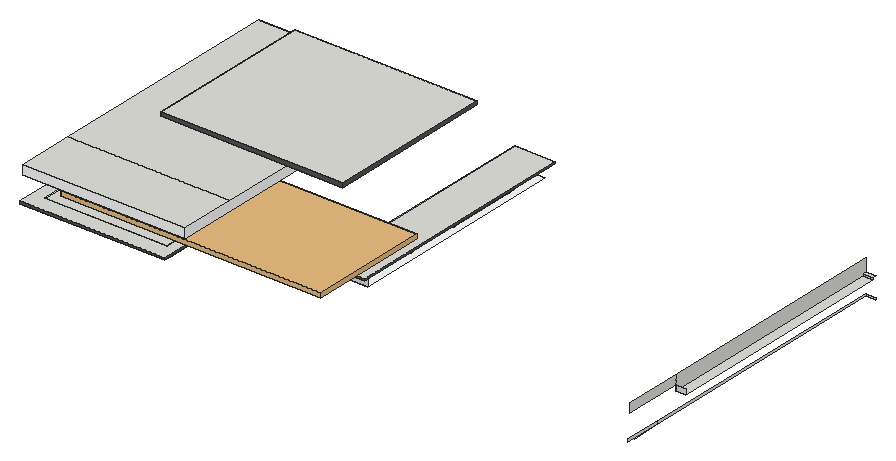
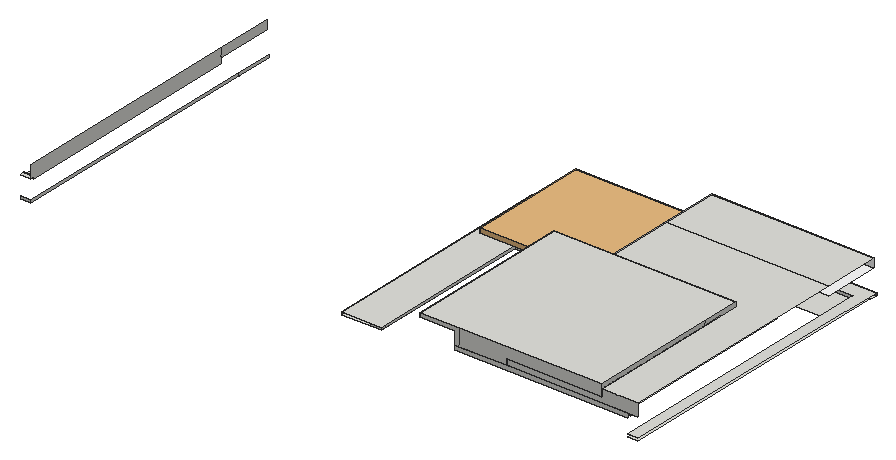
# SketchUp Ruby script. Lengths in inches.
U = 1.inch
M = Sketchup.active_model
def pt(a) = Geom::Point3d.new(a.map { |v| v * U })
def face(e, loops, mat)
  f = e.add_face(loops[0].map { |a| pt(a) })
  loops[1..].each { |l| e.add_face(l.map { |a| pt(a) }).erase! }
  f.material = f.back_material = mat if mat
  f
end
# faces: each face lists its corners as indices into pts; further lists are holes
def faces(e, pts, list, mat = nil) = list.each { |f| face(e, (f[0].is_a?(Array) ? f : [f]).map { |l| l.map { |i| pts[i] } }, mat) }
# xy, xz, yz: faces in a plane at the given z, y or x. An outline is a flat list of corners, or four numbers for a rectangle; further outlines are holes
def ring(l) = l.size == 4 ? [[l[0], l[1]], [l[2], l[1]], [l[2], l[3]], [l[0], l[3]]] : l.each_slice(2).to_a
def flat(e, list, mat, &to3) = list.each { |f| face(e, (f[0].is_a?(Array) ? f : [f]).map { |l| ring(l).map { |u, v| to3.(u, v) } }, mat) }
def xy(e, z, list, mat = nil) = flat(e, list, mat) { |x, y| [x, y, z] }
def xz(e, y, list, mat = nil) = flat(e, list, mat) { |x, z| [x, y, z] }
def yz(e, x, list, mat = nil) = flat(e, list, mat) { |y, z| [x, y, z] }
def lines(e, pts, list) = list.each { |a, b| e.add_line(pt(pts[a]), pt(pts[b])) }
# prism: a flat outline (further loops are holes) pulled along v
def prism(e, loops, v, mat = nil)
  f = face(e, loops, mat); d = Geom::Vector3d.new(v.map { |x| x * U })
  f.pushpull(f.normal.samedirection?(d) ? d.length : -d.length)
end
def box(e, o, s, mat = nil) = prism(e, [[o, [o[0] + s[0], o[1], o[2]], [o[0] + s[0], o[1] + s[1], o[2]], [o[0], o[1] + s[1], o[2]]]], [0, 0, s[2]], mat)
def at(x, y, z, deg = 0) = Geom::Transformation.translation(pt([x, y, z])) * Geom::Transformation.rotation(ORIGIN, Z_AXIS, deg.degrees)
def axes(o, x, y, z) = Geom::Transformation.new([*x, 0, *y, 0, *z, 0, *pt(o).to_a, 1])
def part(name) = M.definitions.add(name)
# library, detail: a bought-in or finely detailed component or shape, given as its bounding box
def library(name, o, s) = part(name).tap { |d| box(d.entities, o, s) }
def detail(e, o, s) = box(e.add_group.entities, o, s)
def put(e, d, t, mat = nil) = e.add_instance(d, t).tap { |i| i.material = mat if mat }
def group(e, t, mat = nil) = e.add_group.tap { |g| g.transformation = t; g.material = mat if mat }.entities
root = M.entities
M.materials.add("[Color M00]").color = [255, 255, 255]
M.materials.add("[Color M06]").color = [86, 86, 86]
c1 = library("Mesh Light\#4",[-0.5,-0.5,-0.1],[1,1,0.2])
c2 = part("Group\#24")
xy(c2.entities,0,[[203.13,95.41,201.58,95.62,200.13,96.22,198.89,97.17,197.9375,98.41,197.34,99.86,197.13,101.41,197.34,102.96,197.9375,104.41,198.89,105.65,200.13,106.61,201.58,107.21,203.13,107.41,204.6875,107.21,206.13,106.61,207.375,105.65,208.33,104.41,208.93,102.96,209.13,101.41,208.93,99.86,208.33,98.41,207.375,97.17,206.13,96.22,204.6875,95.62],[281.57,95.41,280.02,95.62,278.57,96.22,277.33,97.17,276.375,98.41,275.77,99.86,275.57,101.41,275.77,102.96,276.375,104.41,277.33,105.65,278.57,106.61,280.02,107.21,281.57,107.41,283.125,107.21,284.57,106.61,285.8125,105.65,286.77,104.41,287.37,102.96,287.57,101.41,287.37,99.86,286.77,98.41,285.8125,97.17,284.57,96.22,283.125,95.62],[350.95,95.41,349.39,95.62,347.95,96.22,346.7,97.17,345.75,98.41,345.15,99.86,344.95,101.41,345.15,102.96,345.75,104.41,346.7,105.65,347.95,106.61,349.39,107.21,350.95,107.41,352.5,107.21,353.95,106.61,355.1875,105.65,356.14,104.41,356.74,102.96,356.95,101.41,356.74,99.86,356.14,98.41,355.1875,97.17,353.95,96.22,352.5,95.62],[376,162.85,374.44,163.05,373,163.65,371.75,164.6,370.8,165.85,370.2,167.29,370,168.85,370.2,170.4,370.8,171.85,371.75,173.09,373,174.04,374.44,174.64,376,174.85,377.55,174.64,379,174.04,380.24,173.09,381.19,171.85,381.79,170.4,382,168.85,381.79,167.29,381.19,165.85,380.24,164.6,379,163.65,377.55,163.05]],"[Color M00]")
xy(c2.entities,33.4375,[[6,0,4.45,0.2,3,0.8,1.76,1.76,0.8,3,0.2,4.45,0,6,0.2,7.55,0.8,9,1.76,10.24,3,11.2,4.45,11.8,6,12,7.55,11.8,9,11.2,10.24,10.24,11.2,9,11.8,7.55,12,6,11.8,4.45,11.2,3,10.24,1.76,9,0.8,7.55,0.2],[83.125,0,81.57,0.2,80.125,0.8,78.88,1.76,77.93,3,77.33,4.45,77.125,6,77.33,7.55,77.93,9,78.88,10.24,80.125,11.2,81.57,11.8,83.125,12,84.68,11.8,86.125,11.2,87.37,10.24,88.32,9,88.92,7.55,89.125,6,88.92,4.45,88.32,3,87.37,1.76,86.125,0.8,84.68,0.2],[166.6875,0,165.13,0.2,163.6875,0.8,162.44,1.76,161.49,3,160.89,4.45,160.6875,6,160.89,7.55,161.49,9,162.44,10.24,163.6875,11.2,165.13,11.8,166.6875,12,168.24,11.8,169.6875,11.2,170.93,10.24,171.88,9,172.48,7.55,172.6875,6,172.48,4.45,171.88,3,170.93,1.76,169.6875,0.8,168.24,0.2],[166.6875,88.9375,165.13,89.14,163.6875,89.74,162.44,90.69,161.49,91.9375,160.89,93.38,160.6875,94.9375,160.89,96.49,161.49,97.9375,162.44,99.18,163.6875,100.13,165.13,100.73,166.6875,100.9375,168.24,100.73,169.6875,100.13,170.93,99.18,171.88,97.9375,172.48,96.49,172.6875,94.9375,172.48,93.38,171.88,91.9375,170.93,90.69,169.6875,89.74,168.24,89.14]],"[Color M00]")
put(c2.entities,c1,axes([191,87.42,16.72],[382.99758,0,0],[0,175.84579,0],[0,0,34.4375]))
c3 = library("Group\#23",[-0.5,-0.5,-0.1],[13,110.375,0.2])
xy(root,270.375,[[2063.54,581.75,2275.98,592.75],[2064.92,592.75,2064.92,1019,2079.65,1019,2079.65,605.03,2260.47,605.03,2260.47,703.86,2269.48,703.86,2269.48,592.75],[2269.48,592.75,2275.98,636.6875],[2956.13,592.75,2957.51,636.6875],[2079.65,605.03,2260.47,605.03,2260.47,703.86,2256.86,703.86,2256.86,660.21,2079.65,660.21],
  [2269.48,636.6875,2275.98,728.9375],[2256.86,703.86,2269.48,774.3125]])
xy(root,274.0625,[[2063.54,581.75,2275.98,581.75,2275.98,674.36,2269.48,674.36,2269.48,703.86,2260.47,703.86,2260.47,605.03,2079.65,605.03,2079.65,1019,2064.92,1019,2064.92,636.6875,2063.54,636.6875],[2269.48,674.36,2275.98,728.9375]])
xy(root,274.0625,[[[2275.98,674.36,2275.98,728.9375,2459.67,728.9375,2459.67,999.35,2500.29,999.35,2500.29,674.36],[2311.19,696.41,2312.75,696.61,2314.19,697.21,2315.4375,698.17,2316.39,699.41,2316.99,700.86,2317.19,702.41,2316.99,703.96,2316.39,705.41,2315.4375,706.65,2314.19,707.61,2312.75,708.21,2311.19,708.41,2309.64,708.21,2308.19,707.61,2306.95,706.65,2306,705.41,2305.4,703.96,2305.19,702.41,2305.4,700.86,2306,699.41,2306.95,698.17,2308.19,697.21,2309.64,696.61],[2389.63,696.41,2391.19,696.61,2392.63,697.21,2393.875,698.17,2394.83,699.41,2395.43,700.86,2395.63,702.41,2395.43,703.96,2394.83,705.41,2393.875,706.65,2392.63,707.61,2391.19,708.21,2389.63,708.41,2388.08,708.21,2386.63,707.61,2385.39,706.65,2384.4375,705.41,2383.84,703.96,2383.63,702.41,2383.84,700.86,2384.4375,699.41,2385.39,698.17,2386.63,697.21,2388.08,696.61],[2459.01,696.41,2460.56,696.61,2462.01,697.21,2463.25,698.17,2464.2,699.41,2464.8,700.86,2465.01,702.41,2464.8,703.96,2464.2,705.41,2463.25,706.65,2462.01,707.61,2460.56,708.21,2459.01,708.41,2457.45,708.21,2456.01,707.61,2454.76,706.65,2453.8125,705.41,2453.21,703.96,2453.01,702.41,2453.21,700.86,2453.8125,699.41,2454.76,698.17,2456.01,697.21,2457.45,696.61],[2484.06,763.84,2485.61,764.05,2487.06,764.65,2488.3,765.6,2489.26,766.84,2489.86,768.29,2490.06,769.84,2489.86,771.4,2489.26,772.84,2488.3,774.09,2487.06,775.04,2485.61,775.64,2484.06,775.84,2482.51,775.64,2481.06,775.04,2479.82,774.09,2478.86,772.84,2478.26,771.4,2478.06,769.84,2478.26,768.29,2478.86,766.84,2479.82,765.6,2481.06,764.65,2482.51,764.05],[2484.06,844.28,2485.61,844.49,2487.06,845.09,2488.3,846.04,2489.26,847.28,2489.86,848.73,2490.06,850.28,2489.86,851.83,2489.26,853.28,2488.3,854.52,2487.06,855.48,2485.61,856.08,2484.06,856.28,2482.51,856.08,2481.06,855.48,2479.82,854.52,2478.86,853.28,2478.26,851.83,2478.06,850.28,2478.26,848.73,2478.86,847.28,2479.82,846.04,2481.06,845.09,2482.51,844.49],[2484.06,941.66,2485.61,941.86,2487.06,942.46,2488.3,943.41,2489.26,944.66,2489.86,946.1,2490.06,947.66,2489.86,949.21,2489.26,950.66,2488.3,951.9,2487.06,952.85,2485.61,953.45,2484.06,953.66,2482.51,953.45,2481.06,952.85,2479.82,951.9,2478.86,950.66,2478.26,949.21,2478.06,947.66,2478.26,946.1,2478.86,944.66,2479.82,943.41,2481.06,942.46,2482.51,941.86]]],"[Color M00]")
xy(root,283.9375,[[2269.48,668.11,2500.29,674.36],[2269.48,674.36,2269.48,774.3125,2440.84,774.3125,2440.84,1019,2500.29,1019,2500.29,674.36]])
xy(root,287.375,[[2269.48,668.11,2500.29,668.11,2500.29,1019,2440.84,1019,2440.84,774.3125,2269.48,774.3125]])
xy(root,295.8125,[[2089.96,731.45,2089.96,1012.63,2256.86,1012.63,2256.86,852.1875,2247.33,852.1875,2247.33,731.45],[2256.86,852.1875,2327.29,1012.63]])
xy(root,299.625,[[2957.51,668.18,2972.24,1012.63]])
xy(root,302.5625,[[2079.65,1012.63,2256.86,1019],[2256.86,1012.63,2327.29,1019],[2957.51,1012.63,2972.24,1019]])
xy(root,307.5,[[[2064.92,584.86,2064.92,668.18,2079.65,668.18,2079.65,636.86,2256.86,636.86,2256.86,829.8125,2303.29,829.8125,2303.29,584.86],[2274.75,689.9375,2276.3,690.14,2277.75,690.74,2278.99,691.69,2279.95,692.9375,2280.54,694.38,2280.75,695.9375,2280.54,697.49,2279.95,698.9375,2278.99,700.18,2277.75,701.13,2276.3,701.73,2274.75,701.9375,2273.2,701.73,2271.75,701.13,2270.51,700.18,2269.55,698.9375,2268.95,697.49,2268.75,695.9375,2268.95,694.38,2269.55,692.9375,2270.51,691.69,2271.75,690.74,2273.2,690.14],[2274.75,601,2276.3,601.2,2277.75,601.8,2278.99,602.76,2279.95,604,2280.54,605.45,2280.75,607,2280.54,608.55,2279.95,610,2278.99,611.24,2277.75,612.19,2276.3,612.79,2274.75,613,2273.2,612.79,2271.75,612.19,2270.51,611.24,2269.55,610,2268.95,608.55,2268.75,607,2268.95,605.45,2269.55,604,2270.51,602.76,2271.75,601.8,2273.2,601.2],[2114.0625,601,2115.61,601.2,2117.0625,601.8,2118.3,602.76,2119.26,604,2119.86,605.45,2120.0625,607,2119.86,608.55,2119.26,610,2118.3,611.24,2117.0625,612.19,2115.61,612.79,2114.0625,613,2112.51,612.79,2111.0625,612.19,2109.82,611.24,2108.87,610,2108.27,608.55,2108.0625,607,2108.27,605.45,2108.87,604,2109.82,602.76,2111.0625,601.8,2112.51,601.2],[2191.1875,601,2192.74,601.2,2194.1875,601.8,2195.43,602.76,2196.38,604,2196.98,605.45,2197.1875,607,2196.98,608.55,2196.38,610,2195.43,611.24,2194.1875,612.19,2192.74,612.79,2191.1875,613,2189.63,612.79,2188.1875,612.19,2186.94,611.24,2185.99,610,2185.39,608.55,2185.1875,607,2185.39,605.45,2185.99,604,2186.94,602.76,2188.1875,601.8,2189.63,601.2]]],"[Color M00]")
xy(root,310.3125,[[2117.29,829.8125,2256.86,1019]])
xy(root,320.75,[[2064.92,584.86,2303.29,668.18],[2064.92,668.18,2303.29,668.18,2303.29,772.1875,2117.29,772.1875,2117.29,1019,2064.92,1019],[2303.29,772.1875,2303.29,829.8125,2333.29,829.8125,2333.29,1019,2384.86,1019,2384.86,772.1875]])
xy(root,326.5,[[2117.29,772.1875,2384.86,1019]])
xz(root,581.75,[[2063.54,270.375,2275.98,274.0625]],"[Color M06]")
xz(root,584.86,[[2064.92,307.5,2303.29,320.75]],"[Color M00]")
xz(root,605.03,[[2079.65,270.375,2260.47,274.0625]])
xz(root,636.6875,[[2956.13,270.375,2957.51,274.0625]])
xz(root,668.11,[[2269.48,283.9375,2500.29,287.375]],"[Color M06]")
xz(root,668.18,[[2957.51,299.625,2972.24,307.5]])
xz(root,674.36,[[2269.48,274.0625,2500.29,283.9375]])
xz(root,703.86,[[2260.47,270.375,2269.48,274.0625]])
xz(root,772.1875,[[2117.29,320.75,2384.86,326.5]],"[Color M06]")
xz(root,774.3125,[[2269.48,283.9375,2440.84,287.375]])
xz(root,829.8125,[[2256.86,307.5,2303.29,310.3125]])
xz(root,1012.63,[[2079.65,295.8125,2256.86,302.5625],[2256.86,295.8125,2327.29,302.5625],[2957.51,299.625,2972.24,302.5625]])
xz(root,1019,[[2957.51,270.375,2972.24,274.0625],[2440.84,283.9375,2456.54,287.375],[2079.65,295.8125,2333.29,302.5625],[2064.92,302.5625,2064.92,320.75,2117.29,320.75,2117.29,310.3125,2256.86,310.3125,2256.86,302.5625],[2256.86,302.5625,2256.86,310.3125,2117.29,310.3125,2117.29,326.5,2327.29,326.5,2327.29,302.5625],
  [2327.29,302.5625,2327.29,326.5,2384.86,326.5,2384.86,320.75,2333.29,320.75,2333.29,302.5625]])
yz(root,2117.29,[[801.8125,310.3125,829.8125,320.75],[829.8125,310.3125,1019,320.75],[772.1875,320.75,829.8125,326.5],[829.8125,320.75,1019,326.5]])
yz(root,2256.86,[[829.8125,295.8125,1012.63,302.5625],[829.8125,302.5625,1019,310.3125]])
yz(root,2260.47,[[605.03,270.375,703.86,274.0625]])
yz(root,2269.48,[[728.9375,270.375,728.9375,274.0625,674.36,274.0625,674.36,283.9375,774.3125,283.9375,774.3125,270.375],[703.86,270.375,728.9375,274.0625],[668.11,283.9375,774.3125,287.375]])
yz(root,2275.98,[[581.75,270.375,728.9375,274.0625]],"[Color M06]")
yz(root,2303.29,[[584.86,307.5,829.8125,320.75]],"[Color M00]")
yz(root,2384.86,[[772.1875,320.75,1019,326.5]],"[Color M06]")
yz(root,2440.84,[[774.3125,283.9375,1012.63,287.375],[1012.63,283.9375,1019,287.375]])
yz(root,2500.29,[[668.11,283.9375,1019,287.375]],"[Color M06]")
yz(root,2956.13,[[581.75,270.375,636.6875,274.0625]])
yz(root,2957.51,[[636.6875,270.375,1019,274.0625],[668.18,299.625,668.18,320.75,1019,320.75,1019,302.5625,1012.63,302.5625,1012.63,299.625],[584.86,307.5,668.18,320.75]])
p = [[2311.19,696.41,274.0625],[2309.64,696.61,274.0625],[2309.64,696.61,274.75],[2311.19,696.41,274.75],[2312.75,696.61,274.0625],[2312.75,696.61,274.75],
  [2389.63,696.41,274.0625],[2388.08,696.61,274.0625],[2388.08,696.61,274.75],[2389.63,696.41,274.75],[2391.19,696.61,274.0625],[2391.19,696.61,274.75],
  [2459.01,696.41,274.0625],[2457.45,696.61,274.0625],[2457.45,696.61,274.75],[2459.01,696.41,274.75],[2460.56,696.61,274.0625],[2460.56,696.61,274.75],
  [2308.19,697.21,274.0625],[2308.19,697.21,274.75],[2314.19,697.21,274.0625],[2314.19,697.21,274.75],[2386.63,697.21,274.0625],[2386.63,697.21,274.75],
  [2392.63,697.21,274.0625],[2392.63,697.21,274.75],[2456.01,697.21,274.0625],[2456.01,697.21,274.75],[2462.01,697.21,274.0625],[2462.01,697.21,274.75],
  [2306.95,698.17,274.0625],[2306.95,698.17,274.75],[2315.4375,698.17,274.0625],[2315.4375,698.17,274.75],[2385.39,698.17,274.0625],[2385.39,698.17,274.75],
  [2393.875,698.17,274.0625],[2393.875,698.17,274.75],[2454.76,698.17,274.0625],[2454.76,698.17,274.75],[2463.25,698.17,274.0625],[2463.25,698.17,274.75],
  [2306,699.41,274.0625],[2306,699.41,274.75],[2316.39,699.41,274.0625],[2316.39,699.41,274.75],[2384.4375,699.41,274.0625],[2384.4375,699.41,274.75],
  [2394.83,699.41,274.0625],[2394.83,699.41,274.75],[2453.8125,699.41,274.0625],[2453.8125,699.41,274.75],[2464.2,699.41,274.0625],[2464.2,699.41,274.75],
  [2305.4,700.86,274.0625],[2305.4,700.86,274.75],[2316.99,700.86,274.0625],[2316.99,700.86,274.75],[2383.84,700.86,274.0625],[2383.84,700.86,274.75],
  [2395.43,700.86,274.0625],[2395.43,700.86,274.75],[2453.21,700.86,274.0625],[2453.21,700.86,274.75],[2464.8,700.86,274.0625],[2464.8,700.86,274.75],
  [2305.19,702.41,274.0625],[2305.19,702.41,274.75],[2317.19,702.41,274.0625],[2317.19,702.41,274.75],[2383.63,702.41,274.0625],[2383.63,702.41,274.75],
  [2395.63,702.41,274.0625],[2395.63,702.41,274.75],[2453.01,702.41,274.0625],[2453.01,702.41,274.75],[2465.01,702.41,274.0625],[2465.01,702.41,274.75],
  [2305.4,703.96,274.0625],[2305.4,703.96,274.75],[2316.99,703.96,274.0625],[2316.99,703.96,274.75],[2383.84,703.96,274.0625],[2383.84,703.96,274.75],
  [2395.43,703.96,274.0625],[2395.43,703.96,274.75],[2453.21,703.96,274.0625],[2453.21,703.96,274.75],[2464.8,703.96,274.0625],[2464.8,703.96,274.75],
  [2306,705.41,274.0625],[2306,705.41,274.75],[2316.39,705.41,274.0625],[2316.39,705.41,274.75],[2384.4375,705.41,274.0625],[2384.4375,705.41,274.75],
  [2394.83,705.41,274.0625],[2394.83,705.41,274.75],[2453.8125,705.41,274.0625],[2453.8125,705.41,274.75],[2464.2,705.41,274.0625],[2464.2,705.41,274.75],
  [2306.95,706.65,274.0625],[2306.95,706.65,274.75],[2315.4375,706.65,274.0625],[2315.4375,706.65,274.75],[2385.39,706.65,274.0625],[2385.39,706.65,274.75],
  [2393.875,706.65,274.0625],[2393.875,706.65,274.75],[2454.76,706.65,274.0625],[2454.76,706.65,274.75],[2463.25,706.65,274.0625],[2463.25,706.65,274.75],
  [2308.19,707.61,274.0625],[2308.19,707.61,274.75],[2314.19,707.61,274.0625],[2314.19,707.61,274.75],[2386.63,707.61,274.0625],[2386.63,707.61,274.75],
  [2392.63,707.61,274.0625],[2392.63,707.61,274.75],[2456.01,707.61,274.0625],[2456.01,707.61,274.75],[2462.01,707.61,274.0625],[2462.01,707.61,274.75],
  [2309.64,708.21,274.0625],[2309.64,708.21,274.75],[2312.75,708.21,274.0625],[2312.75,708.21,274.75],[2388.08,708.21,274.0625],[2388.08,708.21,274.75],
  [2391.19,708.21,274.0625],[2391.19,708.21,274.75],[2457.45,708.21,274.0625],[2457.45,708.21,274.75],[2460.56,708.21,274.0625],[2460.56,708.21,274.75],
  [2311.19,708.41,274.0625],[2311.19,708.41,274.75],[2389.63,708.41,274.0625],[2389.63,708.41,274.75],[2459.01,708.41,274.0625],[2459.01,708.41,274.75],
  [2484.06,763.84,274.0625],[2482.51,764.05,274.0625],[2482.51,764.05,274.75],[2484.06,763.84,274.75],[2485.61,764.05,274.0625],[2485.61,764.05,274.75],
  [2481.06,764.65,274.0625],[2481.06,764.65,274.75],[2487.06,764.65,274.0625],[2487.06,764.65,274.75],[2479.82,765.6,274.0625],[2479.82,765.6,274.75],
  [2488.3,765.6,274.0625],[2488.3,765.6,274.75],[2478.86,766.84,274.0625],[2478.86,766.84,274.75],[2489.26,766.84,274.0625],[2489.26,766.84,274.75],
  [2478.26,768.29,274.0625],[2478.26,768.29,274.75],[2489.86,768.29,274.0625],[2489.86,768.29,274.75],[2478.06,769.84,274.0625],[2478.06,769.84,274.75],
  [2490.06,769.84,274.0625],[2490.06,769.84,274.75],[2478.26,771.4,274.0625],[2478.26,771.4,274.75],[2489.86,771.4,274.0625],[2489.86,771.4,274.75],
  [2478.86,772.84,274.0625],[2478.86,772.84,274.75],[2489.26,772.84,274.0625],[2489.26,772.84,274.75],[2479.82,774.09,274.0625],[2479.82,774.09,274.75],
  [2488.3,774.09,274.0625],[2488.3,774.09,274.75],[2481.06,775.04,274.0625],[2481.06,775.04,274.75],[2487.06,775.04,274.0625],[2487.06,775.04,274.75],
  [2482.51,775.64,274.0625],[2482.51,775.64,274.75],[2485.61,775.64,274.0625],[2485.61,775.64,274.75],[2484.06,775.84,274.0625],[2484.06,775.84,274.75],
  [2484.06,844.28,274.0625],[2482.51,844.49,274.0625],[2482.51,844.49,274.75],[2484.06,844.28,274.75],[2485.61,844.49,274.0625],[2485.61,844.49,274.75],
  [2481.06,845.09,274.0625],[2481.06,845.09,274.75],[2487.06,845.09,274.0625],[2487.06,845.09,274.75],[2479.82,846.04,274.0625],[2479.82,846.04,274.75],
  [2488.3,846.04,274.0625],[2488.3,846.04,274.75],[2478.86,847.28,274.0625],[2478.86,847.28,274.75],[2489.26,847.28,274.0625],[2489.26,847.28,274.75],
  [2478.26,848.73,274.0625],[2478.26,848.73,274.75],[2489.86,848.73,274.0625],[2489.86,848.73,274.75],[2478.06,850.28,274.0625],[2478.06,850.28,274.75],
  [2490.06,850.28,274.0625],[2490.06,850.28,274.75],[2478.26,851.83,274.0625],[2478.26,851.83,274.75],[2489.86,851.83,274.0625],[2489.86,851.83,274.75],
  [2478.86,853.28,274.0625],[2478.86,853.28,274.75],[2489.26,853.28,274.0625],[2489.26,853.28,274.75],[2479.82,854.52,274.0625],[2479.82,854.52,274.75],
  [2488.3,854.52,274.0625],[2488.3,854.52,274.75],[2481.06,855.48,274.0625],[2481.06,855.48,274.75],[2487.06,855.48,274.0625],[2487.06,855.48,274.75],
  [2482.51,856.08,274.0625],[2482.51,856.08,274.75],[2485.61,856.08,274.0625],[2485.61,856.08,274.75],[2484.06,856.28,274.0625],[2484.06,856.28,274.75],
  [2484.06,941.66,274.0625],[2482.51,941.86,274.0625],[2482.51,941.86,274.75],[2484.06,941.66,274.75],[2485.61,941.86,274.0625],[2485.61,941.86,274.75],
  [2481.06,942.46,274.0625],[2481.06,942.46,274.75],[2487.06,942.46,274.0625],[2487.06,942.46,274.75],[2479.82,943.41,274.0625],[2479.82,943.41,274.75],
  [2488.3,943.41,274.0625],[2488.3,943.41,274.75],[2478.86,944.66,274.0625],[2478.86,944.66,274.75],[2489.26,944.66,274.0625],[2489.26,944.66,274.75],
  [2478.26,946.1,274.0625],[2478.26,946.1,274.75],[2489.86,946.1,274.0625],[2489.86,946.1,274.75],[2478.06,947.66,274.0625],[2478.06,947.66,274.75],
  [2490.06,947.66,274.0625],[2490.06,947.66,274.75],[2478.26,949.21,274.0625],[2478.26,949.21,274.75],[2489.86,949.21,274.0625],[2489.86,949.21,274.75],
  [2478.86,950.66,274.0625],[2478.86,950.66,274.75],[2489.26,950.66,274.0625],[2489.26,950.66,274.75],[2479.82,951.9,274.0625],[2479.82,951.9,274.75],
  [2488.3,951.9,274.0625],[2488.3,951.9,274.75],[2481.06,952.85,274.0625],[2481.06,952.85,274.75],[2487.06,952.85,274.0625],[2487.06,952.85,274.75],
  [2482.51,953.45,274.0625],[2482.51,953.45,274.75],[2485.61,953.45,274.0625],[2485.61,953.45,274.75],[2484.06,953.66,274.0625],[2484.06,953.66,274.75],
  [2114.0625,601,307.5],[2112.51,601.2,307.5],[2112.51,601.2,308.1875],[2114.0625,601,308.1875],[2115.61,601.2,307.5],[2115.61,601.2,308.1875],
  [2191.1875,601,307.5],[2189.63,601.2,307.5],[2189.63,601.2,308.1875],[2191.1875,601,308.1875],[2192.74,601.2,307.5],[2192.74,601.2,308.1875],
  [2274.75,601,307.5],[2273.2,601.2,307.5],[2273.2,601.2,308.1875],[2274.75,601,308.1875],[2276.3,601.2,307.5],[2276.3,601.2,308.1875],
  [2111.0625,601.8,307.5],[2111.0625,601.8,308.1875],[2117.0625,601.8,307.5],[2117.0625,601.8,308.1875],[2188.1875,601.8,307.5],[2188.1875,601.8,308.1875],
  [2194.1875,601.8,307.5],[2194.1875,601.8,308.1875],[2271.75,601.8,307.5],[2271.75,601.8,308.1875],[2277.75,601.8,307.5],[2277.75,601.8,308.1875],
  [2109.82,602.76,307.5],[2109.82,602.76,308.1875],[2118.3,602.76,307.5],[2118.3,602.76,308.1875],[2186.94,602.76,307.5],[2186.94,602.76,308.1875],
  [2195.43,602.76,307.5],[2195.43,602.76,308.1875],[2270.51,602.76,307.5],[2270.51,602.76,308.1875],[2278.99,602.76,307.5],[2278.99,602.76,308.1875],
  [2108.87,604,307.5],[2108.87,604,308.1875],[2119.26,604,307.5],[2119.26,604,308.1875],[2185.99,604,307.5],[2185.99,604,308.1875],
  [2196.38,604,307.5],[2196.38,604,308.1875],[2269.55,604,307.5],[2269.55,604,308.1875],[2279.95,604,307.5],[2279.95,604,308.1875],
  [2108.27,605.45,307.5],[2108.27,605.45,308.1875],[2119.86,605.45,307.5],[2119.86,605.45,308.1875],[2185.39,605.45,307.5],[2185.39,605.45,308.1875],
  [2196.98,605.45,307.5],[2196.98,605.45,308.1875],[2268.95,605.45,307.5],[2268.95,605.45,308.1875],[2280.54,605.45,307.5],[2280.54,605.45,308.1875],
  [2120.0625,607,307.5],[2120.0625,607,308.1875],[2185.1875,607,307.5],[2185.1875,607,308.1875],[2197.1875,607,307.5],[2197.1875,607,308.1875],
  [2268.75,607,307.5],[2268.75,607,308.1875],[2280.75,607,307.5],[2280.75,607,308.1875],[2119.86,608.55,307.5],[2119.86,608.55,308.1875],
  [2185.39,608.55,307.5],[2185.39,608.55,308.1875],[2196.98,608.55,307.5],[2196.98,608.55,308.1875],[2268.95,608.55,307.5],[2268.95,608.55,308.1875],
  [2280.54,608.55,307.5],[2280.54,608.55,308.1875],[2108.27,608.55,307.5],[2108.87,610,307.5],[2108.87,610,308.1875],[2108.27,608.55,308.1875],
  [2119.26,610,307.5],[2119.26,610,308.1875],[2185.99,610,307.5],[2185.99,610,308.1875],[2196.38,610,307.5],[2196.38,610,308.1875],
  [2269.55,610,307.5],[2269.55,610,308.1875],[2279.95,610,307.5],[2279.95,610,308.1875],[2109.82,611.24,307.5],[2109.82,611.24,308.1875],
  [2118.3,611.24,307.5],[2118.3,611.24,308.1875],[2186.94,611.24,307.5],[2186.94,611.24,308.1875],[2195.43,611.24,307.5],[2195.43,611.24,308.1875],
  [2270.51,611.24,307.5],[2270.51,611.24,308.1875],[2278.99,611.24,307.5],[2278.99,611.24,308.1875],[2111.0625,612.19,307.5],[2111.0625,612.19,308.1875],
  [2117.0625,612.19,307.5],[2117.0625,612.19,308.1875],[2188.1875,612.19,307.5],[2188.1875,612.19,308.1875],[2194.1875,612.19,307.5],[2194.1875,612.19,308.1875],
  [2271.75,612.19,307.5],[2271.75,612.19,308.1875],[2277.75,612.19,307.5],[2277.75,612.19,308.1875],[2112.51,612.79,307.5],[2112.51,612.79,308.1875],
  [2115.61,612.79,307.5],[2115.61,612.79,308.1875],[2189.63,612.79,307.5],[2189.63,612.79,308.1875],[2192.74,612.79,307.5],[2192.74,612.79,308.1875],
  [2273.2,612.79,307.5],[2273.2,612.79,308.1875],[2276.3,612.79,307.5],[2276.3,612.79,308.1875],[2114.0625,613,307.5],[2114.0625,613,308.1875],
  [2191.1875,613,307.5],[2191.1875,613,308.1875],[2274.75,613,307.5],[2274.75,613,308.1875],[2274.75,689.9375,307.5],[2273.2,690.14,307.5],
  [2273.2,690.14,308.1875],[2274.75,689.9375,308.1875],[2276.3,690.14,307.5],[2276.3,690.14,308.1875],[2271.75,690.74,307.5],[2271.75,690.74,308.1875],
  [2277.75,690.74,307.5],[2277.75,690.74,308.1875],[2270.51,691.69,307.5],[2270.51,691.69,308.1875],[2278.99,691.69,307.5],[2278.99,691.69,308.1875],
  [2269.55,692.9375,307.5],[2269.55,692.9375,308.1875],[2279.95,692.9375,307.5],[2279.95,692.9375,308.1875],[2268.95,694.38,307.5],[2268.95,694.38,308.1875],
  [2280.54,694.38,307.5],[2280.54,694.38,308.1875],[2268.75,695.9375,307.5],[2268.75,695.9375,308.1875],[2280.75,695.9375,307.5],[2280.75,695.9375,308.1875],
  [2268.95,697.49,307.5],[2268.95,697.49,308.1875],[2280.54,697.49,307.5],[2280.54,697.49,308.1875],[2269.55,698.9375,307.5],[2269.55,698.9375,308.1875],
  [2279.95,698.9375,307.5],[2279.95,698.9375,308.1875],[2270.51,700.18,307.5],[2270.51,700.18,308.1875],[2278.99,700.18,307.5],[2278.99,700.18,308.1875],
  [2271.75,701.13,307.5],[2271.75,701.13,308.1875],[2277.75,701.13,307.5],[2277.75,701.13,308.1875],[2273.2,701.73,307.5],[2273.2,701.73,308.1875],
  [2276.3,701.73,307.5],[2276.3,701.73,308.1875],[2274.75,701.9375,307.5],[2274.75,701.9375,308.1875],[2327.29,1012.63,302.5625],[2327.29,829.8125,302.5625],
  [2327.29,852.1875,295.8125],[2327.29,829.8125,295.8125],[2333.29,852.1875,295.8125],[2256.86,774.3125,270.375],[2256.86,774.3125,282.1875],[2117.29,801.8125,310.3125],
  [2286.92,801.8125,310.3125],[2459.67,999.35,274.0625],[2459.67,999.35,282.1875]]
faces(root,p,[[0,1,2,3],[4,0,3,5],[6,7,8,9],[10,6,9,11],[12,13,14,15],[16,12,15,17],[1,18,19,2],[20,4,5,21],
  [7,22,23,8],[24,10,11,25],[13,26,27,14],[28,16,17,29],[18,30,31,19],[32,20,21,33],[22,34,35,23],[36,24,25,37],
  [26,38,39,27],[40,28,29,41],[30,42,43,31],[44,32,33,45],[34,46,47,35],[48,36,37,49],[38,50,51,39],[52,40,41,53],
  [42,54,55,43],[56,44,45,57],[46,58,59,47],[60,48,49,61],[50,62,63,51],[64,52,53,65],[54,66,67,55],[68,56,57,69],
  [58,70,71,59],[72,60,61,73],[62,74,75,63],[76,64,65,77],[66,78,79,67],[80,68,69,81],[70,82,83,71],[84,72,73,85],
  [74,86,87,75],[88,76,77,89],[78,90,91,79],[92,80,81,93],[82,94,95,83],[96,84,85,97],[86,98,99,87],[100,88,89,101],
  [90,102,103,91],[104,92,93,105],[94,106,107,95],[108,96,97,109],[98,110,111,99],[112,100,101,113],[102,114,115,103],[116,104,105,117],
  [106,118,119,107],[120,108,109,121],[110,122,123,111],[124,112,113,125],[114,126,127,115],[128,116,117,129],[118,130,131,119],[132,120,121,133],
  [122,134,135,123],[136,124,125,137],[126,138,139,127],[138,128,129,139],[130,140,141,131],[140,132,133,141],[134,142,143,135],[142,136,137,143],
  [144,145,146,147],[148,144,147,149],[145,150,151,146],[152,148,149,153],[150,154,155,151],[156,152,153,157],[154,158,159,155],[160,156,157,161],
  [158,162,163,159],[164,160,161,165],[162,166,167,163],[168,164,165,169],[166,170,171,167],[172,168,169,173],[170,174,175,171],[176,172,173,177],
  [174,178,179,175],[180,176,177,181],[178,182,183,179],[184,180,181,185],[182,186,187,183],[188,184,185,189],[186,190,191,187],[190,188,189,191],
  [192,193,194,195],[196,192,195,197],[193,198,199,194],[200,196,197,201],[198,202,203,199],[204,200,201,205],[202,206,207,203],[208,204,205,209],
  [206,210,211,207],[212,208,209,213],[210,214,215,211],[216,212,213,217],[214,218,219,215],[220,216,217,221],[218,222,223,219],[224,220,221,225],
  [222,226,227,223],[228,224,225,229],[226,230,231,227],[232,228,229,233],[230,234,235,231],[236,232,233,237],[234,238,239,235],[238,236,237,239],
  [240,241,242,243],[244,240,243,245],[241,246,247,242],[248,244,245,249],[246,250,251,247],[252,248,249,253],[250,254,255,251],[256,252,253,257],
  [254,258,259,255],[260,256,257,261],[258,262,263,259],[264,260,261,265],[262,266,267,263],[268,264,265,269],[266,270,271,267],[272,268,269,273],
  [270,274,275,271],[276,272,273,277],[274,278,279,275],[280,276,277,281],[278,282,283,279],[284,280,281,285],[282,286,287,283],[286,284,285,287],
  [288,289,290,291],[292,288,291,293],[294,295,296,297],[298,294,297,299],[300,301,302,303],[304,300,303,305],[289,306,307,290],[308,292,293,309],
  [295,310,311,296],[312,298,299,313],[301,314,315,302],[316,304,305,317],[306,318,319,307],[320,308,309,321],[310,322,323,311],[324,312,313,325],
  [314,326,327,315],[328,316,317,329],[318,330,331,319],[332,320,321,333],[322,334,335,323],[336,324,325,337],[326,338,339,327],[340,328,329,341],
  [330,342,343,331],[344,332,333,345],[334,346,347,335],[348,336,337,349],[338,350,351,339],[352,340,341,353],[354,344,345,355],[346,356,357,347],
  [358,348,349,359],[350,360,361,351],[362,352,353,363],[364,354,355,365],[356,366,367,357],[368,358,359,369],[360,370,371,361],[372,362,363,373],
  [374,375,376,377],[378,364,365,379],[366,380,381,367],[382,368,369,383],[370,384,385,371],[386,372,373,387],[375,388,389,376],[390,378,379,391],
  [380,392,393,381],[394,382,383,395],[384,396,397,385],[398,386,387,399],[388,400,401,389],[402,390,391,403],[392,404,405,393],[406,394,395,407],
  [396,408,409,397],[410,398,399,411],[400,412,413,401],[414,402,403,415],[404,416,417,405],[418,406,407,419],[408,420,421,409],[422,410,411,423],
  [412,424,425,413],[424,414,415,425],[416,426,427,417],[426,418,419,427],[420,428,429,421],[428,422,423,429],[430,431,432,433],[434,430,433,435],
  [431,436,437,432],[438,434,435,439],[436,440,441,437],[442,438,439,443],[440,444,445,441],[446,442,443,447],[444,448,449,445],[450,446,447,451],
  [448,452,453,449],[454,450,451,455],[452,456,457,453],[458,454,455,459],[456,460,461,457],[462,458,459,463],[460,464,465,461],[466,462,463,467],
  [464,468,469,465],[470,466,467,471],[468,472,473,469],[474,470,471,475],[472,476,477,473],[476,474,475,477]],"[Color M00]")
lines(root,p,[[478,479],[480,481],[480,482],[483,484],[485,486],[487,488]])
put(root,c2,at(2108.0625,601,274.75))
put(root,c3,at(2478.06,844.28,274.75))
